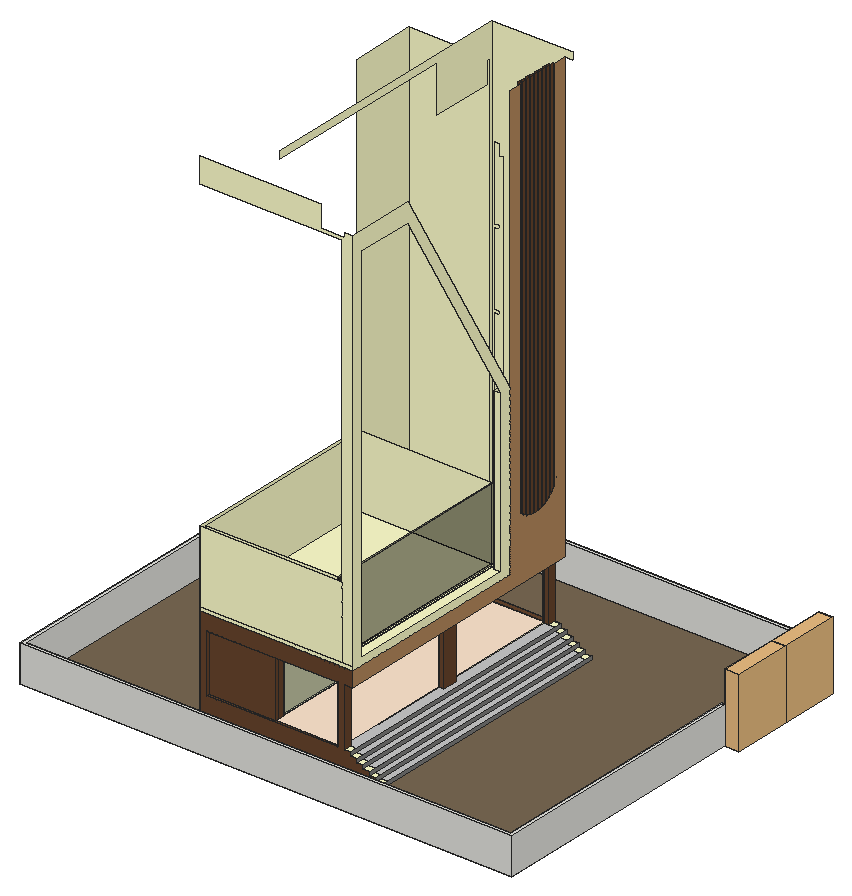
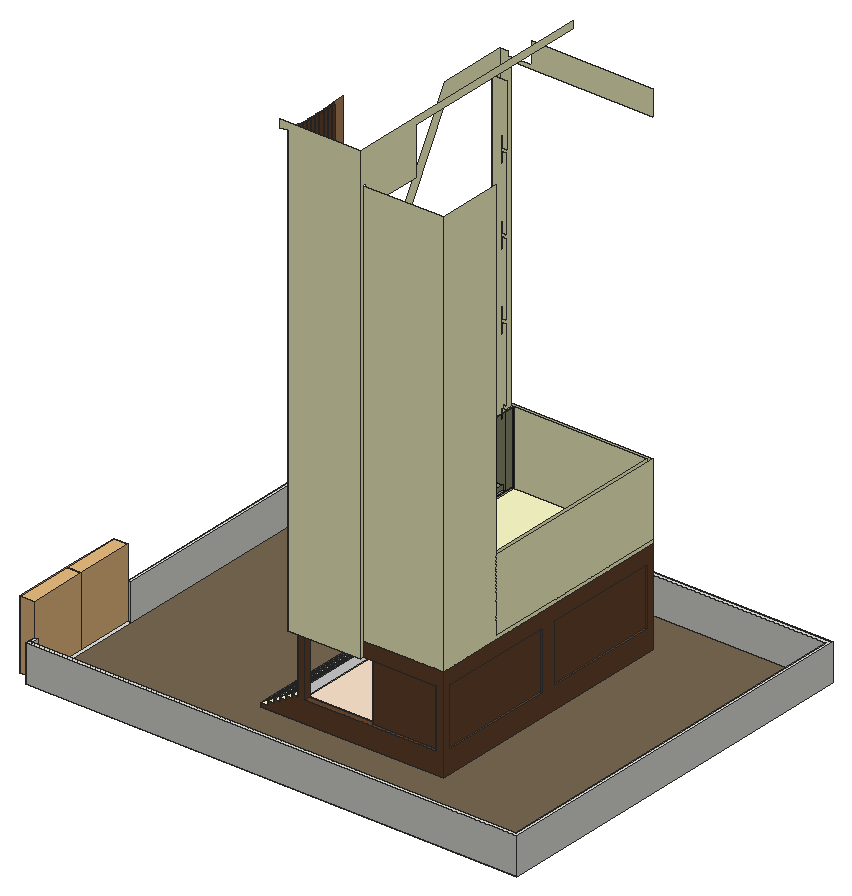
# SketchUp Ruby script. Lengths in inches.
U = 1.inch
M = Sketchup.active_model
def pt(a) = Geom::Point3d.new(a.map { |v| v * U })
def face(e, loops, mat)
  f = e.add_face(loops[0].map { |a| pt(a) })
  loops[1..].each { |l| e.add_face(l.map { |a| pt(a) }).erase! }
  f.material = f.back_material = mat if mat
  f
end
# faces: each face lists its corners as indices into pts; further lists are holes
def faces(e, pts, list, mat = nil) = list.each { |f| face(e, (f[0].is_a?(Array) ? f : [f]).map { |l| l.map { |i| pts[i] } }, mat) }
# xy, xz, yz: faces in a plane at the given z, y or x. An outline is a flat list of corners, or four numbers for a rectangle; further outlines are holes
def ring(l) = l.size == 4 ? [[l[0], l[1]], [l[2], l[1]], [l[2], l[3]], [l[0], l[3]]] : l.each_slice(2).to_a
def flat(e, list, mat, &to3) = list.each { |f| face(e, (f[0].is_a?(Array) ? f : [f]).map { |l| ring(l).map { |u, v| to3.(u, v) } }, mat) }
def xy(e, z, list, mat = nil) = flat(e, list, mat) { |x, y| [x, y, z] }
def xz(e, y, list, mat = nil) = flat(e, list, mat) { |x, z| [x, y, z] }
def yz(e, x, list, mat = nil) = flat(e, list, mat) { |y, z| [x, y, z] }
def lines(e, pts, list) = list.each { |a, b| e.add_line(pt(pts[a]), pt(pts[b])) }
# prism: a flat outline (further loops are holes) pulled along v
def prism(e, loops, v, mat = nil)
  f = face(e, loops, mat); d = Geom::Vector3d.new(v.map { |x| x * U })
  f.pushpull(f.normal.samedirection?(d) ? d.length : -d.length)
end
def box(e, o, s, mat = nil) = prism(e, [[o, [o[0] + s[0], o[1], o[2]], [o[0] + s[0], o[1] + s[1], o[2]], [o[0], o[1] + s[1], o[2]]]], [0, 0, s[2]], mat)
def at(x, y, z, deg = 0) = Geom::Transformation.translation(pt([x, y, z])) * Geom::Transformation.rotation(ORIGIN, Z_AXIS, deg.degrees)
def axes(o, x, y, z) = Geom::Transformation.new([*x, 0, *y, 0, *z, 0, *pt(o).to_a, 1])
def part(name) = M.definitions.add(name)
# library, detail: a bought-in or finely detailed component or shape, given as its bounding box
def library(name, o, s) = part(name).tap { |d| box(d.entities, o, s) }
def detail(e, o, s) = box(e.add_group.entities, o, s)
def put(e, d, t, mat = nil) = e.add_instance(d, t).tap { |i| i.material = mat if mat }
def group(e, t, mat = nil) = e.add_group.tap { |g| g.transformation = t; g.material = mat if mat }.entities
root = M.entities
M.materials.add("C01_Vanilla_Cream").color = [255, 230, 206]
M.materials.add("E01_Mint_Frost").color = [255, 255, 204]
M.materials.add("Glass_Safety_01").color = [0, 0, 0]
M.materials["Glass_Safety_01"].alpha = 0.25
M.materials.add("Glass_Safety_1").color = [78, 90, 94]
M.materials["Glass_Safety_1"].alpha = 0.25
M.materials.add("Plaster_03_1K").color = [121, 105, 83]
M.materials.add("ThomThom - Waistcoat1").color = [201, 201, 201]
M.materials.add("ThomThom - Waistcoat2").color = [127, 127, 126]
M.materials.add("Wood_Floor_01_1K").color = [181, 137, 94]
M.materials.add("Wood_Veneer_15_1K").color = [103, 69, 45]
c1 = library("Ornamental gate leaf",[0,0,0],[161.42,42.43,280.3])
c2 = part("cong")
put(c2.entities,c1,axes([244.78,234.5625,0],[-1,0,0],[0,1,0],[0,0,1]))
put(c2.entities,c1,at(244.78,234.5625,0))
xy(root,-24,[[0,0,0,650.08,809.44,650.08,809.44,632.08,803.44,632.08,803.44,644.08,6,644.08,6,6,803.44,6,803.44,440.08,809.44,440.08,809.44,0],[803.44,440.08,809.44,632.08]])
xy(root,-24,[[235.07,75.71,535.07,507.71]],"C01_Vanilla_Cream")
xy(root,-24,[[6,6,803.44,644.08]],"Plaster_03_1K")
xy(root,-18,[[525.07,75.71,535.07,87.71],[525.07,495.71,535.07,507.71]],"E01_Mint_Frost")
xy(root,-18,[[525.07,87.71,535.07,495.71]],"ThomThom - Waistcoat1")
xy(root,-12,[[515.07,75.71,525.07,87.71],[515.07,495.71,525.07,507.71]],"E01_Mint_Frost")
xy(root,-12,[[515.07,87.71,525.07,495.71]],"ThomThom - Waistcoat1")
xy(root,-6,[[505.07,75.71,515.07,87.71],[505.07,495.71,515.07,507.71]],"E01_Mint_Frost")
xy(root,-6,[[505.07,87.71,515.07,495.71]],"ThomThom - Waistcoat1")
xy(root,0,[[495.07,75.71,505.07,87.71],[495.07,495.71,505.07,507.71]],"E01_Mint_Frost")
xy(root,0,[[495.07,87.71,505.07,495.71]],"ThomThom - Waistcoat1")
xy(root,6,[[485.07,75.71,495.07,87.71],[485.07,495.71,495.07,507.71]],"E01_Mint_Frost")
xy(root,6,[[485.07,87.71,495.07,495.71]],"ThomThom - Waistcoat1")
xy(root,12,[[358.07,80.21,463.07,80.21,463.07,84.71,466.07,84.71,466.07,498.71,358.07,498.71]],"C01_Vanilla_Cream")
xy(root,12,[[475.07,75.71,485.07,87.71],[244.07,84.71,355.07,498.71],[355.07,96.71,358.07,486.71],[235.07,279.71,244.07,303.71],[475.07,495.71,485.07,507.71]],"E01_Mint_Frost")
xy(root,12,[[466.07,87.71,485.07,87.71,485.07,495.71,466.07,495.71,466.07,303.71,475.07,303.71,475.07,279.71,466.07,279.71]],"ThomThom - Waistcoat1")
xy(root,12,[[247.07,75.71,463.07,80.21],[235.07,87.71,239.57,279.71],[235.07,303.71,239.57,495.71],[355.07,498.71,463.07,498.71,463.07,507.71,247.07,507.71,247.07,503.21,355.07,503.21]],"Wood_Veneer_15_1K")
xy(root,36,[[0,0,809.44,0,809.44,440.08,803.44,440.08,803.44,6,6,6,6,644.08,809.44,644.08,809.44,650.08,0,650.08],[803.44,632.08,809.44,644.08]])
xy(root,108,[[475.07,75.71,475.07,507.71,367.07,507.71,367.07,513.71,487.07,513.71,487.07,75.71]],"C01_Vanilla_Cream")
xy(root,108,[[247.07,75.71,247.07,80.21,358.07,80.21,358.07,84.71,463.07,84.71,463.07,75.71],[235.07,87.71,239.57,279.71],[466.07,87.71,475.07,279.71],[235.07,303.71,239.57,495.71],[466.07,303.71,475.07,495.71],
  [355.07,498.71,463.07,507.71],[247.07,503.21,355.07,507.71]],"Wood_Veneer_15_1K")
xy(root,120,[[355.07,96.71,358.07,486.71]],"E01_Mint_Frost")
xy(root,132,[[358.07,84.71,466.07,498.71]],"C01_Vanilla_Cream")
xy(root,132,[[235.07,75.71,475.07,75.71,475.07,156.71,466.07,156.71,466.07,84.71,244.07,84.71,244.07,156.71,235.07,156.71],[244.07,84.71,355.07,498.71],[235.07,156.71,244.07,507.71],[466.07,156.71,475.07,507.71],[244.07,498.71,466.07,507.71]],"E01_Mint_Frost")
xy(root,138,[[235.07,75.71,235.07,399.71,241.07,399.71,241.07,81.71,463.07,81.71,463.07,93.71,469.07,93.71,469.07,75.71],[241.07,81.71,463.07,399.71]],"E01_Mint_Frost")
xy(root,144,[[469.07,93.71,487.07,93.71,487.07,381.71,475.07,381.71,475.07,399.71,469.07,399.71]],"E01_Mint_Frost")
xz(root,0,[[0,-24,809.44,36]])
xz(root,6,[[6,-24,803.44,36]])
xz(root,75.71,[[235.07,132,487.07,138],[235.07,138,469.07,258],[469.07,138,487.07,138,487.07,775,475.07,775,475.07,768,434.72,768,434.72,804,235.07,804,235.07,762,469.07,762]],"E01_Mint_Frost")
xz(root,75.71,[[[235.07,-24,535.07,-24,535.07,-18,525.07,-18,525.07,-12,515.07,-12,515.07,-6,505.07,-6,505.07,0,495.07,0,495.07,6,485.07,6,485.07,12,475.07,12,475.07,108,487.07,108,487.07,132,235.07,132],[247.07,12,463.07,108]]],"Wood_Veneer_15_1K")
xz(root,80.21,[[247.07,12,358.07,108]],"Wood_Veneer_15_1K")
xz(root,81.71,[[241.07,138,458.07,258],[461.07,138,463.07,258]],"E01_Mint_Frost")
xz(root,84.71,[[355.07,12,358.07,108]],"E01_Mint_Frost")
xz(root,84.71,[[244.07,12,355.07,132],[463.07,12,463.07,108,358.07,108,358.07,132,466.07,132,466.07,12],[355.07,108,358.07,132]],"Wood_Veneer_15_1K")
xz(root,87.71,[[466.07,12,475.07,108]],"E01_Mint_Frost")
xz(root,87.71,[[235.07,12,239.57,108]],"Wood_Veneer_15_1K")
xz(root,93.71,[[[463.07,138,463.07,258,469.07,258,469.07,264,463.07,264,463.07,384,469.07,384,469.07,366,471.07,366,471.07,408,469.07,408,469.07,390,463.07,390,463.07,510,469.07,510,469.07,492,471.07,492,471.07,534,469.07,534,469.07,516,463.07,516,463.07,636,469.07,636,469.07,618,471.07,618,471.07,660,469.07,660,469.07,642,461.07,642,461.07,744,487.07,744,487.07,144,469.07,144,469.07,138],[469.07,240,471.07,258]]],"E01_Mint_Frost")
xz(root,96.71,[[355.07,12,358.07,108],[355.07,108,358.07,120]],"E01_Mint_Frost")
xz(root,279.71,[[235.07,12,239.57,108],[466.07,12,475.07,108]],"Wood_Veneer_15_1K")
xz(root,303.71,[[466.07,12,475.07,108]],"E01_Mint_Frost")
xz(root,303.71,[[235.07,12,239.57,108]],"Wood_Veneer_15_1K")
xz(root,381.71,[[475.07,144,487.07,408]],"E01_Mint_Frost")
xz(root,399.71,[[235.07,138,241.07,258],[241.07,138,463.07,258],[463.07,138,469.07,138,469.07,144,475.07,144,475.07,744,469.07,744,469.07,762,463.07,762,463.07,642,469.07,642,469.07,660,471.07,660,471.07,618,469.07,618,469.07,636,463.07,636,463.07,516,469.07,516,469.07,534,471.07,534,471.07,492,469.07,492,469.07,510,463.07,510,463.07,390,469.07,390,469.07,408,471.07,408,471.07,366,469.07,366,469.07,384,463.07,384,463.07,264,469.07,264,469.07,282,471.07,282,471.07,240,469.07,240,469.07,258,463.07,258],[475.07,138,487.07,408]],"E01_Mint_Frost")
xz(root,420,[[485.07,216.27,487.07,233.47],[485.07,233.47,487.07,406.83]],"Wood_Veneer_15_1K")
xz(root,424.21,[[481.07,211.74,485.07,233.53],[481.07,233.53,485.07,406.9]],"Wood_Veneer_15_1K")
xz(root,428.43,[[481.07,208.3,485.07,233.6],[481.07,233.6,485.07,406.96]],"Wood_Veneer_15_1K")
xz(root,432.64,[[481.07,205.63,485.07,233.66],[481.07,233.66,485.07,407.03]],"Wood_Veneer_15_1K")
xz(root,436.86,[[481.07,203.58,485.07,233.73],[481.07,233.73,485.07,407.09]],"Wood_Veneer_15_1K")
xz(root,440.08,[[803.44,-24,809.44,36]])
xz(root,441.07,[[481.07,202.05,485.07,233.79],[481.07,233.79,485.07,407.16]],"Wood_Veneer_15_1K")
xz(root,445.29,[[481.07,200.99,485.07,233.86],[481.07,233.86,485.07,407.22]],"Wood_Veneer_15_1K")
xz(root,449.5,[[481.07,200.36,485.07,233.92],[481.07,233.92,485.07,407.29]],"Wood_Veneer_15_1K")
xz(root,453.71,[[481.07,200.15,485.07,233.99],[481.07,233.99,485.07,407.35]],"Wood_Veneer_15_1K")
xz(root,457.93,[[481.07,200.36,485.07,234.05],[481.07,234.05,485.07,407.42]],"Wood_Veneer_15_1K")
xz(root,462.14,[[481.07,200.99,485.07,234.12],[481.07,234.12,485.07,235.56]],"Wood_Veneer_15_1K")
xz(root,466.36,[[481.07,202.05,485.07,234.18],[481.07,234.18,485.07,407.55]],"Wood_Veneer_15_1K")
xz(root,470.57,[[481.07,203.58,485.07,234.25],[481.07,234.25,485.07,407.61]],"Wood_Veneer_15_1K")
xz(root,474.79,[[481.07,205.63,485.07,234.3125],[481.07,234.3125,485.07,407.68]],"Wood_Veneer_15_1K")
xz(root,479,[[481.07,208.3,485.07,234.38],[481.07,234.38,485.07,407.74]],"Wood_Veneer_15_1K")
xz(root,483.21,[[481.07,211.74,485.07,234.44],[481.07,234.44,485.07,407.81]],"Wood_Veneer_15_1K")
xz(root,486.71,[[355.07,12,358.07,108],[355.07,108,358.07,120]],"E01_Mint_Frost")
xz(root,487.43,[[481.07,216.27,485.07,234.51],[481.07,234.51,485.07,407.87]],"Wood_Veneer_15_1K")
xz(root,491.64,[[485.07,222.51,487.07,234.57],[485.07,234.57,487.07,407.94]],"Wood_Veneer_15_1K")
xz(root,495.71,[[235.07,12,239.57,108],[466.07,12,475.07,108]],"Wood_Veneer_15_1K")
xz(root,498.71,[[244.07,0,466.07,12],[355.07,12,358.07,108]],"E01_Mint_Frost")
xz(root,498.71,[[244.07,12,355.07,132],[463.07,12,466.07,12,466.07,132,358.07,132,358.07,108,463.07,108],[355.07,108,358.07,132]],"Wood_Veneer_15_1K")
xz(root,503.21,[[247.07,12,355.07,108]],"Wood_Veneer_15_1K")
xz(root,507.71,[[466.07,108,475.07,132],[235.07,132,367.07,804]],"E01_Mint_Frost")
xz(root,507.71,[[235.07,-24,235.07,132,367.07,132,367.07,108,247.07,108,247.07,12,463.07,12,463.07,108,475.07,108,475.07,12,485.07,12,485.07,6,495.07,6,495.07,0,505.07,0,505.07,-6,515.07,-6,515.07,-12,525.07,-12,525.07,-18,535.07,-18,535.07,-24],[367.07,108,466.07,132]],"Wood_Veneer_15_1K")
xz(root,513.71,[[367.07,108,367.07,858,499.07,858,499.07,846,487.07,846,487.07,108]],"E01_Mint_Frost")
xz(root,632.08,[[803.44,-24,809.44,36]])
xz(root,644.08,[[6,-24,803.44,36]])
xz(root,650.08,[[0,-24,809.44,36]])
yz(root,0,[[0,-24,650.08,36]])
yz(root,6,[[6,-24,644.08,36]])
yz(root,235.07,[[75.71,132,75.71,138,399.71,138,399.71,804,507.71,804,507.71,132],[75.71,138,399.71,258]],"E01_Mint_Frost")
yz(root,235.07,[[[75.71,-24,507.71,132],[303.71,12,495.71,108],[87.71,12,279.71,108]]],"Wood_Veneer_15_1K")
yz(root,239.57,[[87.71,12,279.71,108],[303.71,12,495.71,108]],"Wood_Veneer_15_1K")
yz(root,241.07,[[81.71,138,399.71,258]],"E01_Mint_Frost")
yz(root,244.07,[[156.71,0,498.71,12]],"E01_Mint_Frost")
yz(root,244.07,[[84.71,12,279.71,132],[279.71,12,498.71,132]],"Wood_Veneer_15_1K")
yz(root,247.07,[[75.71,12,80.21,108],[503.21,12,507.71,108]],"Wood_Veneer_15_1K")
yz(root,355.07,[[84.71,12,84.71,132,498.71,132,498.71,12,486.71,12,486.71,120,96.71,120,96.71,12]],"E01_Mint_Frost")
yz(root,355.07,[[96.71,12,486.71,120]],"Glass_Safety_01")
yz(root,355.07,[[498.71,12,503.21,108]],"Wood_Veneer_15_1K")
yz(root,358.07,[[96.71,12,486.71,120]],"Glass_Safety_1")
yz(root,358.07,[[80.21,12,84.71,108],[84.71,12,96.71,12,96.71,120,486.71,120,486.71,12,498.71,12,498.71,132,84.71,132]],"Wood_Veneer_15_1K")
yz(root,367.07,[[507.71,108,507.71,804,501.71,804,501.71,768,399.71,768,399.71,846,75.71,846,75.71,858,513.71,858,513.71,108]],"E01_Mint_Frost")
yz(root,463.07,[[81.71,138,93.71,258]],"E01_Mint_Frost")
yz(root,463.07,[[75.71,12,84.71,108],[498.71,12,507.71,108]],"Wood_Veneer_15_1K")
yz(root,466.07,[[156.71,0,498.71,12]],"E01_Mint_Frost")
yz(root,466.07,[[84.71,12,84.71,132,279.71,132,279.71,108,87.71,108,87.71,12],[279.71,12,279.71,132,498.71,132,498.71,12,495.71,12,495.71,108,303.71,108,303.71,12]],"Wood_Veneer_15_1K")
yz(root,469.07,[[93.71,138,153.71,144],[153.71,138,399.71,144]],"E01_Mint_Frost")
yz(root,475.07,[[381.71,144,399.71,408]],"E01_Mint_Frost")
yz(root,475.07,[[75.71,12,87.71,108],[279.71,12,303.71,108],[495.71,12,507.71,108]],"Wood_Veneer_15_1K")
yz(root,481.07,[[453.71,200.15,453.71,846,449.5,846,449.5,200.36,451.4,200.21],[457.93,200.36,458.33,200.39,460.625,200.7,462.14,200.99,462.14,846,457.93,846],[445.29,200.99,445.29,846,441.07,846,441.07,202.05,442.28,201.68,444.53,201.13],[466.36,202.05,467.36,202.35,469.53,203.14,470.57,203.58,470.57,846,466.36,846],[436.86,203.58,436.86,846,432.64,846,432.64,205.63,433.68,205.05,435.76,204.04],
  [474.79,205.63,475.77,206.18,477.73,207.41,479,208.3,479,846,474.79,846],[428.43,208.3,428.43,846,424.21,846,424.21,211.74,424.26,211.7,425.99,210.17,427.8125,208.74],[483.21,211.74,484.83,213.3125,486.39,215.02,487.43,216.27,487.43,846,483.21,846]],"Wood_Veneer_15_1K")
yz(root,485.07,[[75.71,6,507.71,12]],"ThomThom - Waistcoat2")
yz(root,485.07,[[453.71,200.15,456.03,200.21,457.93,200.36,457.93,846,453.71,846],[449.5,200.36,449.5,846,445.29,846,445.29,200.99,446.8,200.7,449.1,200.39],[462.14,200.99,462.9,201.13,465.15,201.68,466.36,202.05,466.36,846,462.14,846],[441.07,202.05,441.07,846,436.86,846,436.86,203.58,437.89,203.14,440.07,202.35],[470.57,203.58,471.67,204.04,473.74,205.05,474.79,205.63,474.79,846,470.57,846],
  [432.64,205.63,432.64,846,428.43,846,428.43,208.3,429.7,207.41,431.66,206.18],[479,208.3,479.62,208.74,481.43,210.17,483.17,211.7,483.21,211.74,483.21,846,479,846],[424.21,211.74,424.21,846,420,846,420,216.27,421.03,215.02,422.6,213.3125],[487.43,216.27,487.87,216.8,489.24,218.66,490.52,220.59,491.64,222.51,491.64,846,487.43,846]],"Wood_Veneer_15_1K")
yz(root,487.07,[[[75.71,132,399.71,132,399.71,408,189.71,775,75.71,775],[93.71,144,93.71,744,189.71,744,381.71,408,381.71,144]]],"E01_Mint_Frost")
yz(root,487.07,[[75.71,108,513.71,108,513.71,846,491.64,846,491.64,222.51,490.52,220.59,489.24,218.66,487.87,216.8,487.43,216.27,486.39,215.02,484.83,213.3125,483.21,211.74,483.17,211.7,481.43,210.17,479.62,208.74,479,208.3,477.73,207.41,475.77,206.18,474.79,205.63,473.74,205.05,471.67,204.04,470.57,203.58,469.53,203.14,467.36,202.35,466.36,202.05,465.15,201.68,462.9,201.13,462.14,200.99,460.625,200.7,458.33,200.39,457.93,200.36,456.03,200.21,453.71,200.15,451.4,200.21,449.5,200.36,449.1,200.39,446.8,200.7,445.29,200.99,444.53,201.13,442.28,201.68,441.07,202.05,440.07,202.35,437.89,203.14,436.86,203.58,435.76,204.04,433.68,205.05,432.64,205.63,431.66,206.18,429.7,207.41,428.43,208.3,427.8125,208.74,425.99,210.17,424.26,211.7,424.21,211.74,422.6,213.3125,421.03,215.02,420,216.27,420,846,399.71,846,399.71,132,75.71,132]],"Wood_Floor_01_1K")
yz(root,495.07,[[75.71,0,507.71,6]],"ThomThom - Waistcoat2")
yz(root,505.07,[[75.71,-6,507.71,0]],"ThomThom - Waistcoat2")
yz(root,515.07,[[75.71,-12,507.71,-6]],"ThomThom - Waistcoat2")
yz(root,525.07,[[75.71,-18,507.71,-12]],"ThomThom - Waistcoat2")
yz(root,535.07,[[75.71,-24,507.71,-18]],"ThomThom - Waistcoat2")
yz(root,803.44,[[6,-24,440.08,36],[632.08,-24,644.08,36]])
yz(root,809.44,[[0,-24,440.08,36],[632.08,-24,650.08,36]])
p = [[481.07,453.71,200.15],[481.07,451.4,200.21],[487.07,451.4,200.21],[487.07,453.71,200.15],[485.07,453.71,200.15],[487.07,456.03,200.21],
  [485.07,456.03,200.21],[481.07,449.5,200.36],[485.07,449.5,200.36],[487.07,449.5,200.36],[487.07,457.93,200.36],[485.07,457.93,200.36],
  [487.07,449.1,200.39],[485.07,449.1,200.39],[485.07,446.8,200.7],[487.07,446.8,200.7],[481.07,458.33,200.39],[481.07,457.93,200.36],
  [487.07,458.33,200.39],[481.07,460.625,200.7],[487.07,460.625,200.7],[485.07,445.29,200.99],[487.07,445.29,200.99],[481.07,462.14,200.99],
  [487.07,462.14,200.99],[485.07,462.14,200.99],[481.07,445.29,200.99],[481.07,444.53,201.13],[487.07,444.53,201.13],[487.07,462.9,201.13],
  [485.07,462.9,201.13],[481.07,442.28,201.68],[487.07,442.28,201.68],[487.07,465.15,201.68],[485.07,465.15,201.68],[481.07,441.07,202.05],
  [485.07,441.07,202.05],[487.07,441.07,202.05],[487.07,466.36,202.05],[485.07,466.36,202.05],[485.07,440.07,202.35],[487.07,440.07,202.35],
  [481.07,467.36,202.35],[481.07,466.36,202.05],[487.07,467.36,202.35],[485.07,437.89,203.14],[487.07,437.89,203.14],[481.07,469.53,203.14],
  [487.07,469.53,203.14],[485.07,436.86,203.58],[487.07,436.86,203.58],[481.07,470.57,203.58],[487.07,470.57,203.58],[485.07,470.57,203.58],
  [481.07,436.86,203.58],[481.07,435.76,204.04],[487.07,435.76,204.04],[487.07,471.67,204.04],[485.07,471.67,204.04],[481.07,433.68,205.05],
  [487.07,433.68,205.05],[487.07,473.74,205.05],[485.07,473.74,205.05],[481.07,432.64,205.63],[485.07,432.64,205.63],[487.07,432.64,205.63],
  [487.07,474.79,205.63],[485.07,474.79,205.63],[485.07,431.66,206.18],[487.07,431.66,206.18],[481.07,475.77,206.18],[481.07,474.79,205.63],
  [487.07,475.77,206.18],[485.07,429.7,207.41],[487.07,429.7,207.41],[481.07,477.73,207.41],[487.07,477.73,207.41],[485.07,428.43,208.3],
  [487.07,428.43,208.3],[481.07,479,208.3],[487.07,479,208.3],[485.07,479,208.3],[481.07,428.43,208.3],[481.07,427.8125,208.74],
  [487.07,427.8125,208.74],[487.07,479.62,208.74],[485.07,479.62,208.74],[481.07,425.99,210.17],[487.07,425.99,210.17],[487.07,481.43,210.17],
  [485.07,481.43,210.17],[481.07,424.26,211.7],[487.07,424.26,211.7],[487.07,483.17,211.7],[485.07,483.17,211.7],[487.07,424.21,211.74],
  [485.07,424.21,211.74],[485.07,422.6,213.3125],[487.07,422.6,213.3125],[481.07,424.21,211.74],[481.07,484.83,213.3125],[481.07,483.21,211.74],
  [485.07,483.21,211.74],[487.07,483.21,211.74],[487.07,484.83,213.3125],[485.07,421.03,215.02],[487.07,421.03,215.02],[481.07,486.39,215.02],
  [487.07,486.39,215.02],[485.07,420,216.27],[487.07,420,216.27],[481.07,487.43,216.27],[487.07,487.43,216.27],[485.07,487.43,216.27],
  [487.07,487.87,216.8],[485.07,487.87,216.8],[487.07,489.24,218.66],[485.07,489.24,218.66],[487.07,490.52,220.59],[485.07,490.52,220.59],
  [487.07,491.64,222.51],[485.07,491.64,222.51],[481.07,495.86,138],[481.07,495.86,132],[481.07,415.79,406.77],[481.07,415.79,233.4],
  [481.07,415.79,222.59],[487.07,495.86,233.34],[487.07,495.86,234.64]]
faces(root,p,[[0,1,2,3,4],[5,6,4,3],[1,7,8,9,2],[10,11,6,5],[12,13,14,15],[9,8,13,12],[16,17,11,10,18],[19,16,18,20],
  [15,14,21,22],[23,19,20,24,25],[26,27,28,22,21],[29,30,25,24],[27,31,32,28],[33,34,30,29],[31,35,36,37,32],[38,39,34,33],
  [37,36,40,41],[42,43,39,38,44],[41,40,45,46],[47,42,44,48],[46,45,49,50],[51,47,48,52,53],[54,55,56,50,49],[57,58,53,52],
  [55,59,60,56],[61,62,58,57],[59,63,64,65,60],[66,67,62,61],[65,64,68,69],[70,71,67,66,72],[69,68,73,74],[75,70,72,76],
  [74,73,77,78],[79,75,76,80,81],[82,83,84,78,77],[85,86,81,80],[83,87,88,84],[89,90,86,85],[87,91,92,88],[93,94,90,89],
  [95,96,97,98],[91,99,96,95,92],[100,101,102,103,104],[103,102,94,93],[98,97,105,106],[107,100,104,108],[106,105,109,110],[111,107,108,112,113],
  [114,115,113,112],[116,117,115,114],[118,119,117,116],[120,121,119,118]],"Wood_Veneer_15_1K")
lines(root,p,[[122,123],[124,125],[125,126],[127,128]])
put(root,c2,axes([964.55,388.68,-24],[0,0.5992,0],[-0.56,0,0],[0,0,0.4032]))
g1 = group(root,at(458.07,81.71,138),"Glass_Safety_01")
box(g1,[0,0,0],[3,318,120])
